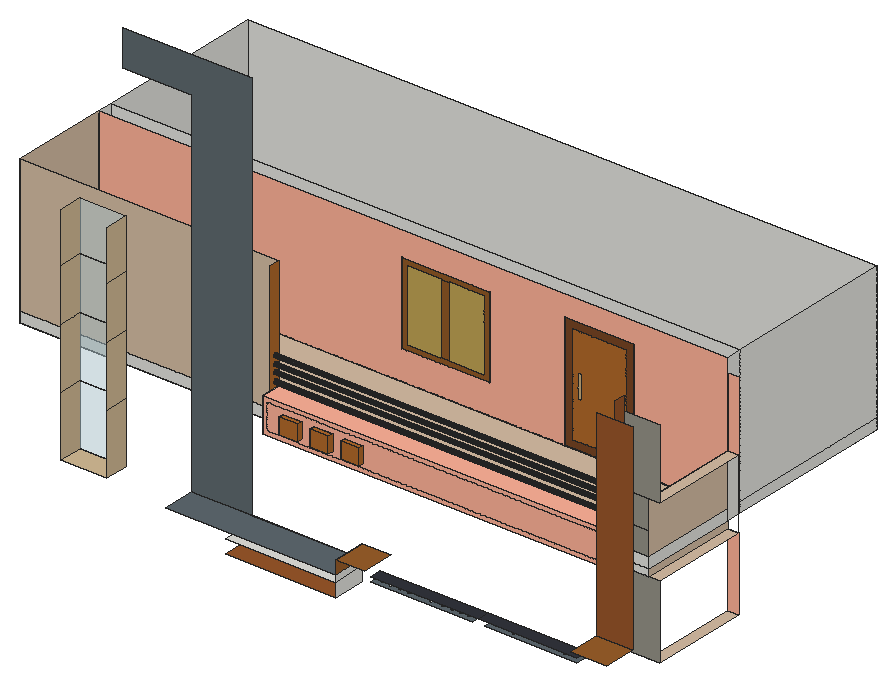
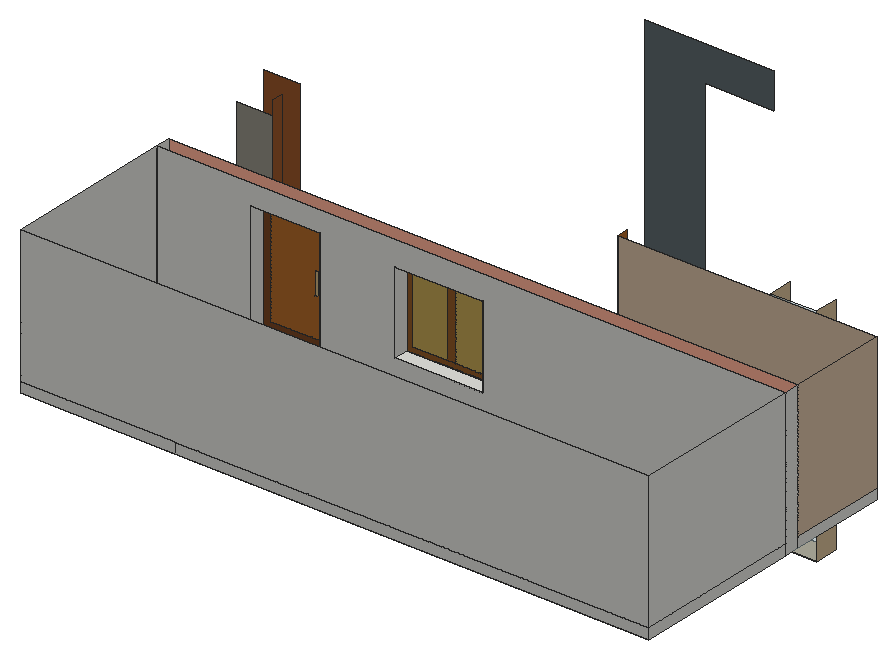
# SketchUp Ruby script. Lengths in inches.
U = 1.inch
M = Sketchup.active_model
def pt(a) = Geom::Point3d.new(a.map { |v| v * U })
def face(e, loops, mat)
  f = e.add_face(loops[0].map { |a| pt(a) })
  loops[1..].each { |l| e.add_face(l.map { |a| pt(a) }).erase! }
  f.material = f.back_material = mat if mat
  f
end
# faces: each face lists its corners as indices into pts; further lists are holes
def faces(e, pts, list, mat = nil) = list.each { |f| face(e, (f[0].is_a?(Array) ? f : [f]).map { |l| l.map { |i| pts[i] } }, mat) }
# xy, xz, yz: faces in a plane at the given z, y or x. An outline is a flat list of corners, or four numbers for a rectangle; further outlines are holes
def ring(l) = l.size == 4 ? [[l[0], l[1]], [l[2], l[1]], [l[2], l[3]], [l[0], l[3]]] : l.each_slice(2).to_a
def flat(e, list, mat, &to3) = list.each { |f| face(e, (f[0].is_a?(Array) ? f : [f]).map { |l| ring(l).map { |u, v| to3.(u, v) } }, mat) }
def xy(e, z, list, mat = nil) = flat(e, list, mat) { |x, y| [x, y, z] }
def xz(e, y, list, mat = nil) = flat(e, list, mat) { |x, z| [x, y, z] }
def yz(e, x, list, mat = nil) = flat(e, list, mat) { |y, z| [x, y, z] }
def lines(e, pts, list) = list.each { |a, b| e.add_line(pt(pts[a]), pt(pts[b])) }
# prism: a flat outline (further loops are holes) pulled along v
def prism(e, loops, v, mat = nil)
  f = face(e, loops, mat); d = Geom::Vector3d.new(v.map { |x| x * U })
  f.pushpull(f.normal.samedirection?(d) ? d.length : -d.length)
end
def box(e, o, s, mat = nil) = prism(e, [[o, [o[0] + s[0], o[1], o[2]], [o[0] + s[0], o[1] + s[1], o[2]], [o[0], o[1] + s[1], o[2]]]], [0, 0, s[2]], mat)
def at(x, y, z, deg = 0) = Geom::Transformation.translation(pt([x, y, z])) * Geom::Transformation.rotation(ORIGIN, Z_AXIS, deg.degrees)
def axes(o, x, y, z) = Geom::Transformation.new([*x, 0, *y, 0, *z, 0, *pt(o).to_a, 1])
def part(name) = M.definitions.add(name)
# library, detail: a bought-in or finely detailed component or shape, given as its bounding box
def library(name, o, s) = part(name).tap { |d| box(d.entities, o, s) }
def detail(e, o, s) = box(e.add_group.entities, o, s)
def put(e, d, t, mat = nil) = e.add_instance(d, t).tap { |i| i.material = mat if mat }
def group(e, t, mat = nil) = e.add_group.tap { |g| g.transformation = t; g.material = mat if mat }.entities
root = M.entities
M.materials.add("[Blinds Cloth Horizontal]").color = [192, 163, 85]
M.materials.add("[Color B02]").color = [255, 178, 153]
M.materials.add("[Color M07]").color = [58, 58, 58]
M.materials.add("[Formica Beige]").color = [211, 187, 149]
M.materials.add("[Formica Graystone]").color = [149, 146, 135]
M.materials.add("[Formica Laminate Dark]").color = [50, 53, 60]
M.materials.add("[Formica Laminate Light]").color = [213, 189, 164]
M.materials.add("[Formica Speckled Grey]").color = [94, 105, 111]
M.materials.add("[Translucent Glass Safety]").color = [204, 235, 244]
M.materials["[Translucent Glass Safety]"].alpha = 0.5
M.materials.add("[Wood Bamboo]").color = [177, 105, 43]
M.materials.add("[Wood Cherry Original]").color = [152, 86, 42]
M.materials.add("[Wood Floor Dark]").color = [153, 94, 42]
M.materials.add("[Wood Floor Light]").color = [204, 176, 127]
M.materials.add("[Wood Floor Parquet]").color = [145, 89, 39]
M.materials.add("[Wood Veneer 01]").color = [120, 70, 37]
xy(root,57.0625,[[221.09,49.81,311.65,57.99]])
xy(root,57.0625,[[221.09,31.06,311.65,49.81]],"[Wood Cherry Original]")
xy(root,60.06,[[65.18,56.99,102.75,76.74]],"[Formica Beige]")
xy(root,62.9375,[[524.83,85.74,533.83,166.38]],"[Formica Laminate Light]")
xy(root,68.21,[[221.09,31.06,311.65,57.99]])
xy(root,73.875,[[172.2,31.06,311.65,57.99]],"[Formica Speckled Grey]")
xy(root,73.98,[[448.68,41.58,448.94,41.61,449.18,41.71,449.39,41.875,449.55,42.08,449.65,42.32,449.68,42.58,449.65,42.84,449.55,43.08,449.39,43.29,449.18,43.45,448.94,43.55,448.68,43.58,448.43,43.55,448.18,43.45,447.98,43.29,447.82,43.08,447.72,42.84,447.68,42.58,447.72,42.32,447.82,42.08,447.98,41.875,448.18,41.71,448.43,41.61]])
xy(root,74.1,[[341.18,41.58,341.44,41.61,341.68,41.71,341.89,41.875,342.05,42.08,342.15,42.32,342.18,42.58,342.15,42.84,342.05,43.08,341.89,43.29,341.68,43.45,341.44,43.55,341.18,43.58,340.93,43.55,340.68,43.45,340.48,43.29,340.32,43.08,340.22,42.84,340.18,42.58,340.22,42.32,340.32,42.08,340.48,41.875,340.68,41.71,340.93,41.61],[348,41.58,348.26,41.61,348.5,41.71,348.7,41.875,348.86,42.08,348.96,42.32,349,42.58,348.96,42.84,348.86,43.08,348.7,43.29,348.5,43.45,348.26,43.55,348,43.58,347.74,43.55,347.5,43.45,347.29,43.29,347.13,43.08,347.03,42.84,347,42.58,347.03,42.32,347.13,42.08,347.29,41.875,347.5,41.71,347.74,41.61],[355.87,41.58,356.13,41.61,356.37,41.71,356.58,41.875,356.74,42.08,356.84,42.32,356.87,42.58,356.84,42.84,356.74,43.08,356.58,43.29,356.37,43.45,356.13,43.55,355.87,43.58,355.61,43.55,355.37,43.45,355.16,43.29,355.01,43.08,354.91,42.84,354.87,42.58,354.91,42.32,355.01,42.08,355.16,41.875,355.37,41.71,355.61,41.61],[363,41.58,363.26,41.61,363.5,41.71,363.7,41.875,363.86,42.08,363.96,42.32,364,42.58,363.96,42.84,363.86,43.08,363.7,43.29,363.5,43.45,363.26,43.55,363,43.58,362.74,43.55,362.5,43.45,362.29,43.29,362.13,43.08,362.03,42.84,362,42.58,362.03,42.32,362.13,42.08,362.29,41.875,362.5,41.71,362.74,41.61],[371.93,41.58,372.19,41.61,372.43,41.71,372.64,41.875,372.8,42.08,372.9,42.32,372.93,42.58,372.9,42.84,372.8,43.08,372.64,43.29,372.43,43.45,372.19,43.55,371.93,43.58,371.68,43.55,371.43,43.45,371.23,43.29,371.07,43.08,370.97,42.84,370.93,42.58,370.97,42.32,371.07,42.08,371.23,41.875,371.43,41.71,371.68,41.61],
  [381.12,41.58,381.38,41.61,381.62,41.71,381.83,41.875,381.99,42.08,382.09,42.32,382.12,42.58,382.09,42.84,381.99,43.08,381.83,43.29,381.62,43.45,381.38,43.55,381.12,43.58,380.86,43.55,380.62,43.45,380.41,43.29,380.26,43.08,380.16,42.84,380.12,42.58,380.16,42.32,380.26,42.08,380.41,41.875,380.62,41.71,380.86,41.61],[390.81,41.58,391.07,41.61,391.31,41.71,391.52,41.875,391.68,42.08,391.77,42.32,391.81,42.58,391.77,42.84,391.68,43.08,391.52,43.29,391.31,43.45,391.07,43.55,390.81,43.58,390.55,43.55,390.31,43.45,390.1,43.29,389.94,43.08,389.84,42.84,389.81,42.58,389.84,42.32,389.94,42.08,390.1,41.875,390.31,41.71,390.55,41.61],[398.25,41.58,398.51,41.61,398.75,41.71,398.95,41.875,399.11,42.08,399.21,42.32,399.25,42.58,399.21,42.84,399.11,43.08,398.95,43.29,398.75,43.45,398.51,43.55,398.25,43.58,397.99,43.55,397.75,43.45,397.54,43.29,397.38,43.08,397.28,42.84,397.25,42.58,397.28,42.32,397.38,42.08,397.54,41.875,397.75,41.71,397.99,41.61],[405.56,41.58,405.82,41.61,406.06,41.71,406.27,41.875,406.43,42.08,406.52,42.32,406.56,42.58,406.52,42.84,406.43,43.08,406.27,43.29,406.06,43.45,405.82,43.55,405.56,43.58,405.3,43.55,405.06,43.45,404.85,43.29,404.69,43.08,404.59,42.84,404.56,42.58,404.59,42.32,404.69,42.08,404.85,41.875,405.06,41.71,405.3,41.61],[412.31,41.58,412.57,41.61,412.81,41.71,413.02,41.875,413.18,42.08,413.27,42.32,413.31,42.58,413.27,42.84,413.18,43.08,413.02,43.29,412.81,43.45,412.57,43.55,412.31,43.58,412.05,43.55,411.81,43.45,411.6,43.29,411.44,43.08,411.34,42.84,411.31,42.58,411.34,42.32,411.44,42.08,411.6,41.875,411.81,41.71,412.05,41.61],
  [435,41.58,435.26,41.61,435.5,41.71,435.7,41.875,435.86,42.08,435.96,42.32,436,42.58,435.96,42.84,435.86,43.08,435.7,43.29,435.5,43.45,435.26,43.55,435,43.58,434.74,43.55,434.5,43.45,434.29,43.29,434.13,43.08,434.03,42.84,434,42.58,434.03,42.32,434.13,42.08,434.29,41.875,434.5,41.71,434.74,41.61],[441.37,41.58,441.63,41.61,441.87,41.71,442.08,41.875,442.24,42.08,442.34,42.32,442.37,42.58,442.34,42.84,442.24,43.08,442.08,43.29,441.87,43.45,441.63,43.55,441.37,43.58,441.11,43.55,440.87,43.45,440.66,43.29,440.51,43.08,440.41,42.84,440.37,42.58,440.41,42.32,440.51,42.08,440.66,41.875,440.87,41.71,441.11,41.61],[448.68,41.58,448.94,41.61,449.18,41.71,449.39,41.875,449.55,42.08,449.65,42.32,449.68,42.58,449.65,42.84,449.55,43.08,449.39,43.29,449.18,43.45,448.94,43.55,448.68,43.58,448.43,43.55,448.18,43.45,447.98,43.29,447.82,43.08,447.72,42.84,447.68,42.58,447.72,42.32,447.82,42.08,447.98,41.875,448.18,41.71,448.43,41.61],[456.56,41.58,456.82,41.61,457.06,41.71,457.27,41.875,457.43,42.08,457.52,42.32,457.56,42.58,457.52,42.84,457.43,43.08,457.27,43.29,457.06,43.45,456.82,43.55,456.56,43.58,456.3,43.55,456.06,43.45,455.85,43.29,455.69,43.08,455.59,42.84,455.56,42.58,455.59,42.32,455.69,42.08,455.85,41.875,456.06,41.71,456.3,41.61],[464.37,41.58,464.63,41.61,464.87,41.71,465.08,41.875,465.24,42.08,465.34,42.32,465.37,42.58,465.34,42.84,465.24,43.08,465.08,43.29,464.87,43.45,464.63,43.55,464.37,43.58,464.11,43.55,463.87,43.45,463.66,43.29,463.51,43.08,463.41,42.84,463.37,42.58,463.41,42.32,463.51,42.08,463.66,41.875,463.87,41.71,464.11,41.61],
  [473.68,41.58,473.94,41.61,474.18,41.71,474.39,41.875,474.55,42.08,474.65,42.32,474.68,42.58,474.65,42.84,474.55,43.08,474.39,43.29,474.18,43.45,473.94,43.55,473.68,43.58,473.43,43.55,473.18,43.45,472.98,43.29,472.82,43.08,472.72,42.84,472.68,42.58,472.72,42.32,472.82,42.08,472.98,41.875,473.18,41.71,473.43,41.61],[483,41.58,483.26,41.61,483.5,41.71,483.7,41.875,483.86,42.08,483.96,42.32,484,42.58,483.96,42.84,483.86,43.08,483.7,43.29,483.5,43.45,483.26,43.55,483,43.58,482.74,43.55,482.5,43.45,482.29,43.29,482.13,43.08,482.03,42.84,482,42.58,482.03,42.32,482.13,42.08,482.29,41.875,482.5,41.71,482.74,41.61],[490.75,41.58,491.01,41.61,491.25,41.71,491.45,41.875,491.61,42.08,491.71,42.32,491.75,42.58,491.71,42.84,491.61,43.08,491.45,43.29,491.25,43.45,491.01,43.55,490.75,43.58,490.49,43.55,490.25,43.45,490.04,43.29,489.88,43.08,489.78,42.84,489.75,42.58,489.78,42.32,489.88,42.08,490.04,41.875,490.25,41.71,490.49,41.61],[497.93,41.58,498.19,41.61,498.43,41.71,498.64,41.875,498.8,42.08,498.9,42.32,498.93,42.58,498.9,42.84,498.8,43.08,498.64,43.29,498.43,43.45,498.19,43.55,497.93,43.58,497.68,43.55,497.43,43.45,497.23,43.29,497.07,43.08,496.97,42.84,496.93,42.58,496.97,42.32,497.07,42.08,497.23,41.875,497.43,41.71,497.68,41.61]])
xy(root,74.1,[[[335.09,37.79,418.54,47.28],[341.18,41.58,341.44,41.61,341.68,41.71,341.89,41.875,342.05,42.08,342.15,42.32,342.18,42.58,342.15,42.84,342.05,43.08,341.89,43.29,341.68,43.45,341.44,43.55,341.18,43.58,340.93,43.55,340.68,43.45,340.48,43.29,340.32,43.08,340.22,42.84,340.18,42.58,340.22,42.32,340.32,42.08,340.48,41.875,340.68,41.71,340.93,41.61],[412.31,41.58,412.57,41.61,412.81,41.71,413.02,41.875,413.18,42.08,413.27,42.32,413.31,42.58,413.27,42.84,413.18,43.08,413.02,43.29,412.81,43.45,412.57,43.55,412.31,43.58,412.05,43.55,411.81,43.45,411.6,43.29,411.44,43.08,411.34,42.84,411.31,42.58,411.34,42.32,411.44,42.08,411.6,41.875,411.81,41.71,412.05,41.61],[348,41.58,348.26,41.61,348.5,41.71,348.7,41.875,348.86,42.08,348.96,42.32,349,42.58,348.96,42.84,348.86,43.08,348.7,43.29,348.5,43.45,348.26,43.55,348,43.58,347.74,43.55,347.5,43.45,347.29,43.29,347.13,43.08,347.03,42.84,347,42.58,347.03,42.32,347.13,42.08,347.29,41.875,347.5,41.71,347.74,41.61],[405.56,41.58,405.82,41.61,406.06,41.71,406.27,41.875,406.43,42.08,406.52,42.32,406.56,42.58,406.52,42.84,406.43,43.08,406.27,43.29,406.06,43.45,405.82,43.55,405.56,43.58,405.3,43.55,405.06,43.45,404.85,43.29,404.69,43.08,404.59,42.84,404.56,42.58,404.59,42.32,404.69,42.08,404.85,41.875,405.06,41.71,405.3,41.61],[355.87,41.58,356.13,41.61,356.37,41.71,356.58,41.875,356.74,42.08,356.84,42.32,356.87,42.58,356.84,42.84,356.74,43.08,356.58,43.29,356.37,43.45,356.13,43.55,355.87,43.58,355.61,43.55,355.37,43.45,355.16,43.29,355.01,43.08,354.91,42.84,354.87,42.58,354.91,42.32,355.01,42.08,355.16,41.875,355.37,41.71,355.61,41.61],[398.25,41.58,398.51,41.61,398.75,41.71,398.95,41.875,399.11,42.08,399.21,42.32,399.25,42.58,399.21,42.84,399.11,43.08,398.95,43.29,398.75,43.45,398.51,43.55,398.25,43.58,397.99,43.55,397.75,43.45,397.54,43.29,397.38,43.08,397.28,42.84,397.25,42.58,397.28,42.32,397.38,42.08,397.54,41.875,397.75,41.71,397.99,41.61],[363,41.58,363.26,41.61,363.5,41.71,363.7,41.875,363.86,42.08,363.96,42.32,364,42.58,363.96,42.84,363.86,43.08,363.7,43.29,363.5,43.45,363.26,43.55,363,43.58,362.74,43.55,362.5,43.45,362.29,43.29,362.13,43.08,362.03,42.84,362,42.58,362.03,42.32,362.13,42.08,362.29,41.875,362.5,41.71,362.74,41.61],[390.81,41.58,391.07,41.61,391.31,41.71,391.52,41.875,391.68,42.08,391.77,42.32,391.81,42.58,391.77,42.84,391.68,43.08,391.52,43.29,391.31,43.45,391.07,43.55,390.81,43.58,390.55,43.55,390.31,43.45,390.1,43.29,389.94,43.08,389.84,42.84,389.81,42.58,389.84,42.32,389.94,42.08,390.1,41.875,390.31,41.71,390.55,41.61],[371.93,41.58,372.19,41.61,372.43,41.71,372.64,41.875,372.8,42.08,372.9,42.32,372.93,42.58,372.9,42.84,372.8,43.08,372.64,43.29,372.43,43.45,372.19,43.55,371.93,43.58,371.68,43.55,371.43,43.45,371.23,43.29,371.07,43.08,370.97,42.84,370.93,42.58,370.97,42.32,371.07,42.08,371.23,41.875,371.43,41.71,371.68,41.61],[381.12,41.58,381.38,41.61,381.62,41.71,381.83,41.875,381.99,42.08,382.09,42.32,382.12,42.58,382.09,42.84,381.99,43.08,381.83,43.29,381.62,43.45,381.38,43.55,381.12,43.58,380.86,43.55,380.62,43.45,380.41,43.29,380.26,43.08,380.16,42.84,380.12,42.58,380.16,42.32,380.26,42.08,380.41,41.875,380.62,41.71,380.86,41.61]],[[428.66,37.79,504.33,47.28],[497.93,41.58,498.19,41.61,498.43,41.71,498.64,41.875,498.8,42.08,498.9,42.32,498.93,42.58,498.9,42.84,498.8,43.08,498.64,43.29,498.43,43.45,498.19,43.55,497.93,43.58,497.68,43.55,497.43,43.45,497.23,43.29,497.07,43.08,496.97,42.84,496.93,42.58,496.97,42.32,497.07,42.08,497.23,41.875,497.43,41.71,497.68,41.61],[441.37,41.58,441.63,41.61,441.87,41.71,442.08,41.875,442.24,42.08,442.34,42.32,442.37,42.58,442.34,42.84,442.24,43.08,442.08,43.29,441.87,43.45,441.63,43.55,441.37,43.58,441.11,43.55,440.87,43.45,440.66,43.29,440.51,43.08,440.41,42.84,440.37,42.58,440.41,42.32,440.51,42.08,440.66,41.875,440.87,41.71,441.11,41.61],[490.75,41.58,491.01,41.61,491.25,41.71,491.45,41.875,491.61,42.08,491.71,42.32,491.75,42.58,491.71,42.84,491.61,43.08,491.45,43.29,491.25,43.45,491.01,43.55,490.75,43.58,490.49,43.55,490.25,43.45,490.04,43.29,489.88,43.08,489.78,42.84,489.75,42.58,489.78,42.32,489.88,42.08,490.04,41.875,490.25,41.71,490.49,41.61],[448.68,41.58,448.94,41.61,449.18,41.71,449.39,41.875,449.55,42.08,449.65,42.32,449.68,42.58,449.65,42.84,449.55,43.08,449.39,43.29,449.18,43.45,448.94,43.55,448.68,43.58,448.43,43.55,448.18,43.45,447.98,43.29,447.82,43.08,447.72,42.84,447.68,42.58,447.72,42.32,447.82,42.08,447.98,41.875,448.18,41.71,448.43,41.61],[483,41.58,483.26,41.61,483.5,41.71,483.7,41.875,483.86,42.08,483.96,42.32,484,42.58,483.96,42.84,483.86,43.08,483.7,43.29,483.5,43.45,483.26,43.55,483,43.58,482.74,43.55,482.5,43.45,482.29,43.29,482.13,43.08,482.03,42.84,482,42.58,482.03,42.32,482.13,42.08,482.29,41.875,482.5,41.71,482.74,41.61],[456.56,41.58,456.82,41.61,457.06,41.71,457.27,41.875,457.43,42.08,457.52,42.32,457.56,42.58,457.52,42.84,457.43,43.08,457.27,43.29,457.06,43.45,456.82,43.55,456.56,43.58,456.3,43.55,456.06,43.45,455.85,43.29,455.69,43.08,455.59,42.84,455.56,42.58,455.59,42.32,455.69,42.08,455.85,41.875,456.06,41.71,456.3,41.61],[473.68,41.58,473.94,41.61,474.18,41.71,474.39,41.875,474.55,42.08,474.65,42.32,474.68,42.58,474.65,42.84,474.55,43.08,474.39,43.29,474.18,43.45,473.94,43.55,473.68,43.58,473.43,43.55,473.18,43.45,472.98,43.29,472.82,43.08,472.72,42.84,472.68,42.58,472.72,42.32,472.82,42.08,472.98,41.875,473.18,41.71,473.43,41.61],[464.37,41.58,464.63,41.61,464.87,41.71,465.08,41.875,465.24,42.08,465.34,42.32,465.37,42.58,465.34,42.84,465.24,43.08,465.08,43.29,464.87,43.45,464.63,43.55,464.37,43.58,464.11,43.55,463.87,43.45,463.66,43.29,463.51,43.08,463.41,42.84,463.37,42.58,463.41,42.32,463.51,42.08,463.66,41.875,463.87,41.71,464.11,41.61],[435,41.58,435.26,41.61,435.5,41.71,435.7,41.875,435.86,42.08,435.96,42.32,436,42.58,435.96,42.84,435.86,43.08,435.7,43.29,435.5,43.45,435.26,43.55,435,43.58,434.74,43.55,434.5,43.45,434.29,43.29,434.13,43.08,434.03,42.84,434,42.58,434.03,42.32,434.13,42.08,434.29,41.875,434.5,41.71,434.74,41.61]]],"[Formica Speckled Grey]")
xy(root,77.6875,[[335.09,37.79,423.6,47.28],[423.6,37.79,504.33,47.28]],"[Formica Laminate Dark]")
xy(root,84.875,[[311.65,31.06,335.09,57.99],[504.33,31.06,533.83,57.99]],"[Wood Floor Dark]")
xy(root,123.3125,[[524.83,85.74,533.83,166.38]],"[Formica Laminate Light]")
xy(root,129,[[9,166.38,398.15,178.72],[398.15,166.38,524.83,178.72],[9,178.72,398.15,319.17],[398.15,178.72,524.83,319.17]])
xy(root,129,[[221.09,68.99,504.33,85.74],[9,85.74,524.83,166.38]],"[Color B02]")
xy(root,136.21,[[238.17,64.74,253.24,68.99],[263.49,64.74,278.55,68.99],[288.61,64.74,303.67,68.99]],"[Wood Bamboo]")
xy(root,137.5,[[391.28,166.38,447.72,178.72],[9,178.72,524.83,319.17]])
xy(root,137.5,[[9,85.74,524.83,166.38]],"[Formica Laminate Light]")
xy(root,149.27,[[238.17,64.74,253.24,68.99],[263.49,64.74,278.55,68.99],[288.61,64.74,303.67,68.99]],"[Wood Bamboo]")
xy(root,157,[[221.09,68.99,504.33,85.74]],"[Color B02]")
xy(root,161.63,[[257.7,166.38,329.95,178.72]])
xy(root,180.5625,[[524.83,85.74,533.83,166.38]],"[Formica Laminate Light]")
xz(root,57.99,[[221.09,57.0625,311.65,68.21],[221.09,68.21,311.65,73.875],[172.2,73.875,221.09,73.875,221.09,395.1875,115.05,395.1875,115.05,365.9375,172.2,365.9375]],"[Formica Speckled Grey]")
xz(root,57.99,[[504.33,84.875,533.83,249]],"[Wood Cherry Original]")
xz(root,64.74,[[238.17,136.21,253.24,149.27],[263.49,136.21,278.55,149.27],[288.61,136.21,303.67,149.27]],"[Wood Bamboo]")
xz(root,68.99,[[238.17,136.21,253.24,149.27],[263.49,136.21,278.55,149.27],[288.61,136.21,303.67,149.27]])
xz(root,68.99,[[[221.09,129,504.33,157],[224.35,132.25,501.08,153.75]],[[224.35,132.25,501.08,153.75],[238.17,136.21,253.24,149.27],[263.49,136.21,278.55,149.27],[288.61,136.21,303.67,149.27]]],"[Color B02]")
xz(root,76.74,[[65.18,60.06,102.75,109.75],[65.18,109.75,102.75,159.44],[65.18,159.44,102.75,203.04],[65.18,203.04,102.75,244.12]],"[Translucent Glass Safety]")
xz(root,85.74,[[504.33,123.3125,524.83,129],[9,129,221.09,137.5],[221.09,129,524.83,137.5]])
xz(root,85.74,[[504.33,62.9375,533.83,123.3125],[221.09,137.5,524.83,157],[504.33,157,524.83,180.5625],[504.33,180.5625,533.83,237.86]],"[Formica Graystone]")
xz(root,85.74,[[9,137.5,221.09,249]],"[Formica Laminate Light]")
xz(root,166.38,[[9,129,524.83,137.5]])
xz(root,166.38,[[262.45,166.38,289.625,224.2],[296.63,166.38,325.2,224.2]],"[Blinds Cloth Horizontal]")
xz(root,166.38,[[524.83,62.9375,533.83,123.3125],[[9,137.5,391.28,137.5,391.28,232,447.72,232,447.72,137.5,524.83,137.5,524.83,249,9,249],[257.7,161.63,329.95,228.95]],[524.83,180.5625,533.83,237.86]],"[Color B02]")
xz(root,166.38,[[[397.83,144.04,441.18,225.46],[401.86,175.28,405.36,194.72]]],"[Wood Bamboo]")
xz(root,166.38,[[401.86,175.28,405.36,194.72]],"[Wood Floor Light]")
xz(root,166.38,[[[257.7,161.63,329.95,228.95],[262.45,166.38,325.2,224.2]],[289.625,166.38,296.63,224.2]],"[Wood Floor Parquet]")
xz(root,166.38,[[[391.28,137.5,447.72,232],[397.83,144.04,441.18,225.46]]],"[Wood Veneer 01]")
xz(root,178.72,[[9,129,524.83,137.5],[[9,137.5,9,249,524.83,249,524.83,137.5,447.72,137.5,447.72,232,391.28,232,391.28,137.5],[257.7,161.63,329.95,228.95]]])
xz(root,319.17,[[9,129,398.15,137.5],[398.15,129,524.83,137.5],[9,137.5,524.83,249]])
yz(root,9,[[85.74,129,166.38,137.5],[166.38,129,178.72,249],[178.72,129,319.17,137.5],[178.72,137.5,319.17,249]])
yz(root,9,[[85.74,137.5,166.38,249]],"[Formica Laminate Light]")
yz(root,65.18,[[56.99,60.06,76.74,109.75],[56.99,109.75,76.74,159.44],[56.99,159.44,76.74,203.04],[56.99,203.04,76.74,244.12]],"[Formica Beige]")
yz(root,102.75,[[56.99,60.06,76.74,109.75],[56.99,109.75,76.74,159.44],[56.99,159.44,76.74,203.04],[56.99,203.04,76.74,244.12]],"[Formica Beige]")
yz(root,221.09,[[68.99,129,76.74,157],[76.74,129,85.74,157]])
yz(root,221.09,[[[76.74,157,85.74,249],[81.3,180.02,80.93,180.07,80.58,180.22,80.29,180.44,80.06,180.74,79.91,181.09,79.87,181.46,79.91,181.83,80.06,182.18,80.29,182.48,80.58,182.71,80.93,182.85,81.3,182.9,81.68,182.85,82.02,182.71,82.32,182.48,82.55,182.18,82.69,181.83,82.74,181.46,82.69,181.09,82.55,180.74,82.32,180.44,82.02,180.22,81.68,180.07],[81.3,173.84,80.93,173.89,80.58,174.03,80.29,174.26,80.06,174.56,79.91,174.9,79.87,175.27,79.91,175.65,80.06,175.99,80.29,176.29,80.58,176.52,80.93,176.66,81.3,176.71,81.68,176.66,82.02,176.52,82.32,176.29,82.55,175.99,82.69,175.65,82.74,175.27,82.69,174.9,82.55,174.56,82.32,174.26,82.02,174.03,81.68,173.89],[81.3,167.96,80.93,168.01,80.58,168.15,80.29,168.38,80.06,168.68,79.91,169.03,79.87,169.4,79.91,169.77,80.06,170.12,80.29,170.42,80.58,170.64,80.93,170.79,81.3,170.84,81.68,170.79,82.02,170.64,82.32,170.42,82.55,170.12,82.69,169.77,82.74,169.4,82.69,169.03,82.55,168.68,82.32,168.38,82.02,168.15,81.68,168.01],[81.3,160.77,80.93,160.82,80.58,160.97,80.29,161.19,80.06,161.49,79.91,161.84,79.87,162.21,79.91,162.58,80.06,162.93,80.29,163.23,80.58,163.46,80.93,163.6,81.3,163.65,81.68,163.6,82.02,163.46,82.32,163.23,82.55,162.93,82.69,162.58,82.74,162.21,82.69,161.84,82.55,161.49,82.32,161.19,82.02,160.97,81.68,160.82]]],"[Wood Bamboo]")
yz(root,238.17,[[64.74,136.21,68.99,149.27]],"[Wood Bamboo]")
yz(root,253.24,[[64.74,136.21,68.99,149.27]],"[Wood Bamboo]")
yz(root,257.7,[[166.38,161.63,178.72,228.95]])
yz(root,263.49,[[64.74,136.21,68.99,149.27]],"[Wood Bamboo]")
yz(root,278.55,[[64.74,136.21,68.99,149.27]],"[Wood Bamboo]")
yz(root,288.61,[[64.74,136.21,68.99,149.27]],"[Wood Bamboo]")
yz(root,303.67,[[64.74,136.21,68.99,149.27]],"[Wood Bamboo]")
yz(root,311.65,[[31.06,57.0625,57.99,68.21],[31.06,68.21,57.99,73.875]])
yz(root,311.65,[[31.06,73.875,57.99,84.875]],"[Wood Floor Dark]")
yz(root,329.95,[[166.38,161.63,178.72,228.95]])
yz(root,391.28,[[166.38,137.5,178.72,232]])
yz(root,447.72,[[166.38,137.5,178.72,232]])
yz(root,504.33,[[68.99,129,76.74,157],[81.3,160.77,81.68,160.82,82.02,160.97,82.32,161.19,82.55,161.49,82.69,161.84,82.74,162.21,82.69,162.58,82.55,162.93,82.32,163.23,82.02,163.46,81.68,163.6,81.3,163.65,80.93,163.6,80.58,163.46,80.29,163.23,80.06,162.93,79.91,162.58,79.87,162.21,79.91,161.84,80.06,161.49,80.29,161.19,80.58,160.97,80.93,160.82],[81.3,167.96,81.68,168.01,82.02,168.15,82.32,168.38,82.55,168.68,82.69,169.03,82.74,169.4,82.69,169.77,82.55,170.12,82.32,170.42,82.02,170.64,81.68,170.79,81.3,170.84,80.93,170.79,80.58,170.64,80.29,170.42,80.06,170.12,79.91,169.77,79.87,169.4,79.91,169.03,80.06,168.68,80.29,168.38,80.58,168.15,80.93,168.01],[81.3,173.84,81.68,173.89,82.02,174.03,82.32,174.26,82.55,174.56,82.69,174.9,82.74,175.27,82.69,175.65,82.55,175.99,82.32,176.29,82.02,176.52,81.68,176.66,81.3,176.71,80.93,176.66,80.58,176.52,80.29,176.29,80.06,175.99,79.91,175.65,79.87,175.27,79.91,174.9,80.06,174.56,80.29,174.26,80.58,174.03,80.93,173.89],[81.3,180.02,81.68,180.07,82.02,180.22,82.32,180.44,82.55,180.74,82.69,181.09,82.74,181.46,82.69,181.83,82.55,182.18,82.32,182.48,82.02,182.71,81.68,182.85,81.3,182.9,80.93,182.85,80.58,182.71,80.29,182.48,80.06,182.18,79.91,181.83,79.87,181.46,79.91,181.09,80.06,180.74,80.29,180.44,80.58,180.22,80.93,180.07]])
yz(root,504.33,[[[76.74,157,85.74,249],[81.3,180.02,81.68,180.07,82.02,180.22,82.32,180.44,82.55,180.74,82.69,181.09,82.74,181.46,82.69,181.83,82.55,182.18,82.32,182.48,82.02,182.71,81.68,182.85,81.3,182.9,80.93,182.85,80.58,182.71,80.29,182.48,80.06,182.18,79.91,181.83,79.87,181.46,79.91,181.09,80.06,180.74,80.29,180.44,80.58,180.22,80.93,180.07],[81.3,160.77,81.68,160.82,82.02,160.97,82.32,161.19,82.55,161.49,82.69,161.84,82.74,162.21,82.69,162.58,82.55,162.93,82.32,163.23,82.02,163.46,81.68,163.6,81.3,163.65,80.93,163.6,80.58,163.46,80.29,163.23,80.06,162.93,79.91,162.58,79.87,162.21,79.91,161.84,80.06,161.49,80.29,161.19,80.58,160.97,80.93,160.82],[81.3,167.96,81.68,168.01,82.02,168.15,82.32,168.38,82.55,168.68,82.69,169.03,82.74,169.4,82.69,169.77,82.55,170.12,82.32,170.42,82.02,170.64,81.68,170.79,81.3,170.84,80.93,170.79,80.58,170.64,80.29,170.42,80.06,170.12,79.91,169.77,79.87,169.4,79.91,169.03,80.06,168.68,80.29,168.38,80.58,168.15,80.93,168.01],[81.3,173.84,81.68,173.89,82.02,174.03,82.32,174.26,82.55,174.56,82.69,174.9,82.74,175.27,82.69,175.65,82.55,175.99,82.32,176.29,82.02,176.52,81.68,176.66,81.3,176.71,80.93,176.66,80.58,176.52,80.29,176.29,80.06,175.99,79.91,175.65,79.87,175.27,79.91,174.9,80.06,174.56,80.29,174.26,80.58,174.03,80.93,173.89]]],"[Wood Cherry Original]")
yz(root,504.46,[[81.3,160.77,81.68,160.82,82.02,160.97,82.32,161.19,82.55,161.49,82.69,161.84,82.74,162.21,82.69,162.58,82.55,162.93,82.32,163.23,82.02,163.46,81.68,163.6,81.3,163.65,80.93,163.6,80.58,163.46,80.29,163.23,80.06,162.93,79.91,162.58,79.87,162.21,79.91,161.84,80.06,161.49,80.29,161.19,80.58,160.97,80.93,160.82]])
yz(root,524.83,[[85.74,129,166.38,137.5],[166.38,129,178.72,249],[178.72,129,319.17,137.5],[178.72,137.5,319.17,249]])
yz(root,524.83,[[85.74,123.3125,166.38,129],[85.74,137.5,166.38,180.5625]],"[Formica Laminate Light]")
p = [[448.43,41.61,74.1],[448.18,41.71,74.1],[448.18,41.71,73.98],[448.43,41.61,73.98],[448.68,41.58,74.1],[448.68,41.58,73.98],
  [448.94,41.61,74.1],[448.94,41.61,73.98],[449.18,41.71,74.1],[449.18,41.71,73.98],[447.98,41.875,74.1],[447.98,41.875,73.98],
  [449.39,41.875,74.1],[449.39,41.875,73.98],[447.82,42.08,74.1],[447.82,42.08,73.98],[449.55,42.08,74.1],[449.55,42.08,73.98],
  [447.72,42.32,74.1],[447.72,42.32,73.98],[449.65,42.32,74.1],[449.65,42.32,73.98],[447.68,42.58,74.1],[447.68,42.58,73.98],
  [449.68,42.58,74.1],[449.68,42.58,73.98],[447.72,42.84,74.1],[447.72,42.84,73.98],[449.65,42.84,74.1],[449.65,42.84,73.98],
  [447.82,43.08,74.1],[447.82,43.08,73.98],[449.55,43.08,74.1],[449.55,43.08,73.98],[447.98,43.29,74.1],[447.98,43.29,73.98],
  [449.39,43.29,74.1],[449.39,43.29,73.98],[448.18,43.45,74.1],[448.18,43.45,73.98],[449.18,43.45,74.1],[449.18,43.45,73.98],
  [448.43,43.55,74.1],[448.43,43.55,73.98],[448.94,43.55,74.1],[448.94,43.55,73.98],[448.68,43.58,74.1],[448.68,43.58,73.98],
  [504.33,80.93,160.82],[504.33,80.58,160.97],[221.09,80.58,160.97],[221.09,80.93,160.82],[504.46,80.93,160.82],[504.46,80.58,160.97],
  [504.33,81.3,160.77],[221.09,81.3,160.77],[504.46,81.3,160.77],[504.33,81.68,160.82],[221.09,81.68,160.82],[504.46,81.68,160.82],
  [504.33,82.02,160.97],[221.09,82.02,160.97],[504.46,82.02,160.97],[504.33,80.29,161.19],[221.09,80.29,161.19],[504.46,80.29,161.19],
  [504.33,82.32,161.19],[221.09,82.32,161.19],[504.46,82.32,161.19],[504.33,80.06,161.49],[221.09,80.06,161.49],[504.46,80.06,161.49],
  [504.33,82.55,161.49],[221.09,82.55,161.49],[504.46,82.55,161.49],[504.33,79.91,161.84],[221.09,79.91,161.84],[504.46,79.91,161.84],
  [504.33,82.69,161.84],[221.09,82.69,161.84],[504.46,82.69,161.84],[504.33,79.87,162.21],[221.09,79.87,162.21],[504.46,79.87,162.21],
  [504.33,82.74,162.21],[221.09,82.74,162.21],[504.46,82.74,162.21],[504.33,79.91,162.58],[221.09,79.91,162.58],[504.46,79.91,162.58],
  [504.33,82.69,162.58],[221.09,82.69,162.58],[504.46,82.69,162.58],[504.33,80.06,162.93],[221.09,80.06,162.93],[504.46,80.06,162.93],
  [504.33,82.55,162.93],[221.09,82.55,162.93],[504.46,82.55,162.93],[504.33,80.29,163.23],[221.09,80.29,163.23],[504.46,80.29,163.23],
  [504.33,82.32,163.23],[221.09,82.32,163.23],[504.46,82.32,163.23],[504.33,80.58,163.46],[221.09,80.58,163.46],[504.46,80.58,163.46],
  [504.33,82.02,163.46],[221.09,82.02,163.46],[504.46,82.02,163.46],[504.33,80.93,163.6],[221.09,80.93,163.6],[504.46,80.93,163.6],
  [504.33,81.68,163.6],[221.09,81.68,163.6],[504.46,81.68,163.6],[504.33,81.3,163.65],[221.09,81.3,163.65],[504.46,81.3,163.65],
  [504.33,80.93,168.01],[504.33,80.58,168.15],[221.09,80.58,168.15],[221.09,80.93,168.01],[504.33,81.3,167.96],[221.09,81.3,167.96],
  [504.33,81.68,168.01],[221.09,81.68,168.01],[504.33,82.02,168.15],[221.09,82.02,168.15],[504.33,80.29,168.38],[221.09,80.29,168.38],
  [504.33,82.32,168.38],[221.09,82.32,168.38],[504.33,80.06,168.68],[221.09,80.06,168.68],[504.33,82.55,168.68],[221.09,82.55,168.68],
  [504.33,79.91,169.03],[221.09,79.91,169.03],[504.33,82.69,169.03],[221.09,82.69,169.03],[504.33,79.87,169.4],[221.09,79.87,169.4],
  [504.33,82.74,169.4],[221.09,82.74,169.4],[504.33,79.91,169.77],[221.09,79.91,169.77],[504.33,82.69,169.77],[221.09,82.69,169.77],
  [504.33,80.06,170.12],[221.09,80.06,170.12],[504.33,82.55,170.12],[221.09,82.55,170.12],[504.33,80.29,170.42],[221.09,80.29,170.42],
  [504.33,82.32,170.42],[221.09,82.32,170.42],[504.33,80.58,170.64],[221.09,80.58,170.64],[504.33,82.02,170.64],[221.09,82.02,170.64],
  [504.33,80.93,170.79],[221.09,80.93,170.79],[504.33,81.68,170.79],[221.09,81.68,170.79],[504.33,81.3,170.84],[221.09,81.3,170.84],
  [504.33,81.3,173.84],[504.33,80.93,173.89],[221.09,80.93,173.89],[221.09,81.3,173.84],[504.33,81.68,173.89],[221.09,81.68,173.89],
  [504.33,80.58,174.03],[221.09,80.58,174.03],[504.33,82.02,174.03],[221.09,82.02,174.03],[504.33,80.29,174.26],[221.09,80.29,174.26],
  [504.33,82.32,174.26],[221.09,82.32,174.26],[504.33,80.06,174.56],[221.09,80.06,174.56],[504.33,82.55,174.56],[221.09,82.55,174.56],
  [504.33,79.91,174.9],[221.09,79.91,174.9],[504.33,82.69,174.9],[221.09,82.69,174.9],[504.33,79.87,175.27],[221.09,79.87,175.27],
  [504.33,82.74,175.27],[221.09,82.74,175.27],[504.33,79.91,175.65],[221.09,79.91,175.65],[504.33,82.69,175.65],[221.09,82.69,175.65],
  [504.33,80.06,175.99],[221.09,80.06,175.99],[504.33,82.55,175.99],[221.09,82.55,175.99],[504.33,80.29,176.29],[221.09,80.29,176.29],
  [504.33,82.32,176.29],[221.09,82.32,176.29],[504.33,80.58,176.52],[221.09,80.58,176.52],[504.33,82.02,176.52],[221.09,82.02,176.52],
  [504.33,80.93,176.66],[221.09,80.93,176.66],[504.33,81.68,176.66],[221.09,81.68,176.66],[504.33,81.3,176.71],[221.09,81.3,176.71],
  [504.33,81.3,180.02],[504.33,80.93,180.07],[221.09,80.93,180.07],[221.09,81.3,180.02],[504.33,81.68,180.07],[221.09,81.68,180.07],
  [504.33,80.58,180.22],[221.09,80.58,180.22],[504.33,82.02,180.22],[221.09,82.02,180.22],[504.33,80.29,180.44],[221.09,80.29,180.44],
  [504.33,82.32,180.44],[221.09,82.32,180.44],[504.33,80.06,180.74],[221.09,80.06,180.74],[504.33,82.55,180.74],[221.09,82.55,180.74],
  [504.33,79.91,181.09],[221.09,79.91,181.09],[504.33,82.69,181.09],[221.09,82.69,181.09],[504.33,79.87,181.46],[221.09,79.87,181.46],
  [504.33,82.74,181.46],[221.09,82.74,181.46],[504.33,79.91,181.83],[221.09,79.91,181.83],[504.33,82.69,181.83],[221.09,82.69,181.83],
  [504.33,80.06,182.18],[221.09,80.06,182.18],[504.33,82.55,182.18],[221.09,82.55,182.18],[504.33,80.29,182.48],[221.09,80.29,182.48],
  [504.33,82.32,182.48],[221.09,82.32,182.48],[504.33,80.58,182.71],[221.09,80.58,182.71],[504.33,82.02,182.71],[221.09,82.02,182.71],
  [504.33,80.93,182.85],[221.09,80.93,182.85],[504.33,81.68,182.85],[221.09,81.68,182.85],[504.33,81.3,182.9],[221.09,81.3,182.9],
  [533.83,166.38,123.3125],[533.83,166.38,180.5625]]
faces(root,p,[[0,1,2,3],[4,0,3,5],[6,4,5,7],[8,6,7,9],[1,10,11,2],[12,8,9,13],[10,14,15,11],[16,12,13,17],
  [14,18,19,15],[20,16,17,21],[18,22,23,19],[24,20,21,25],[22,26,27,23],[28,24,25,29],[26,30,31,27],[32,28,29,33],
  [30,34,35,31],[36,32,33,37],[34,38,39,35],[40,36,37,41],[38,42,43,39],[44,40,41,45],[42,46,47,43],[46,44,45,47],
  [49,48,52,53],[48,54,56,52],[54,57,59,56],[57,60,62,59],[63,49,53,65],[60,66,68,62],[69,63,65,71],[66,72,74,68],
  [75,69,71,77],[72,78,80,74],[81,75,77,83],[78,84,86,80],[87,81,83,89],[84,90,92,86],[93,87,89,95],[90,96,98,92],
  [99,93,95,101],[96,102,104,98],[105,99,101,107],[102,108,110,104],[111,105,107,113],[108,114,116,110],[117,111,113,119],[114,117,119,116]])
faces(root,p,[[48,49,50,51],[54,48,51,55],[57,54,55,58],[60,57,58,61],[49,63,64,50],[66,60,61,67],[63,69,70,64],[72,66,67,73],
  [69,75,76,70],[78,72,73,79],[75,81,82,76],[84,78,79,85],[81,87,88,82],[90,84,85,91],[87,93,94,88],[96,90,91,97],
  [93,99,100,94],[102,96,97,103],[99,105,106,100],[108,102,103,109],[105,111,112,106],[114,108,109,115],[111,117,118,112],[117,114,115,118],
  [120,121,122,123],[124,120,123,125],[126,124,125,127],[128,126,127,129],[121,130,131,122],[132,128,129,133],[130,134,135,131],[136,132,133,137],
  [134,138,139,135],[140,136,137,141],[138,142,143,139],[144,140,141,145],[142,146,147,143],[148,144,145,149],[146,150,151,147],[152,148,149,153],
  [150,154,155,151],[156,152,153,157],[154,158,159,155],[160,156,157,161],[158,162,163,159],[164,160,161,165],[162,166,167,163],[166,164,165,167],
  [168,169,170,171],[172,168,171,173],[169,174,175,170],[176,172,173,177],[174,178,179,175],[180,176,177,181],[178,182,183,179],[184,180,181,185],
  [182,186,187,183],[188,184,185,189],[186,190,191,187],[192,188,189,193],[190,194,195,191],[196,192,193,197],[194,198,199,195],[200,196,197,201],
  [198,202,203,199],[204,200,201,205],[202,206,207,203],[208,204,205,209],[206,210,211,207],[212,208,209,213],[210,214,215,211],[214,212,213,215],
  [216,217,218,219],[220,216,219,221],[217,222,223,218],[224,220,221,225],[222,226,227,223],[228,224,225,229],[226,230,231,227],[232,228,229,233],
  [230,234,235,231],[236,232,233,237],[234,238,239,235],[240,236,237,241],[238,242,243,239],[244,240,241,245],[242,246,247,243],[248,244,245,249],
  [246,250,251,247],[252,248,249,253],[250,254,255,251],[256,252,253,257],[254,258,259,255],[260,256,257,261],[258,262,263,259],[262,260,261,263]],"[Color M07]")
lines(root,p,[[264,265]])
